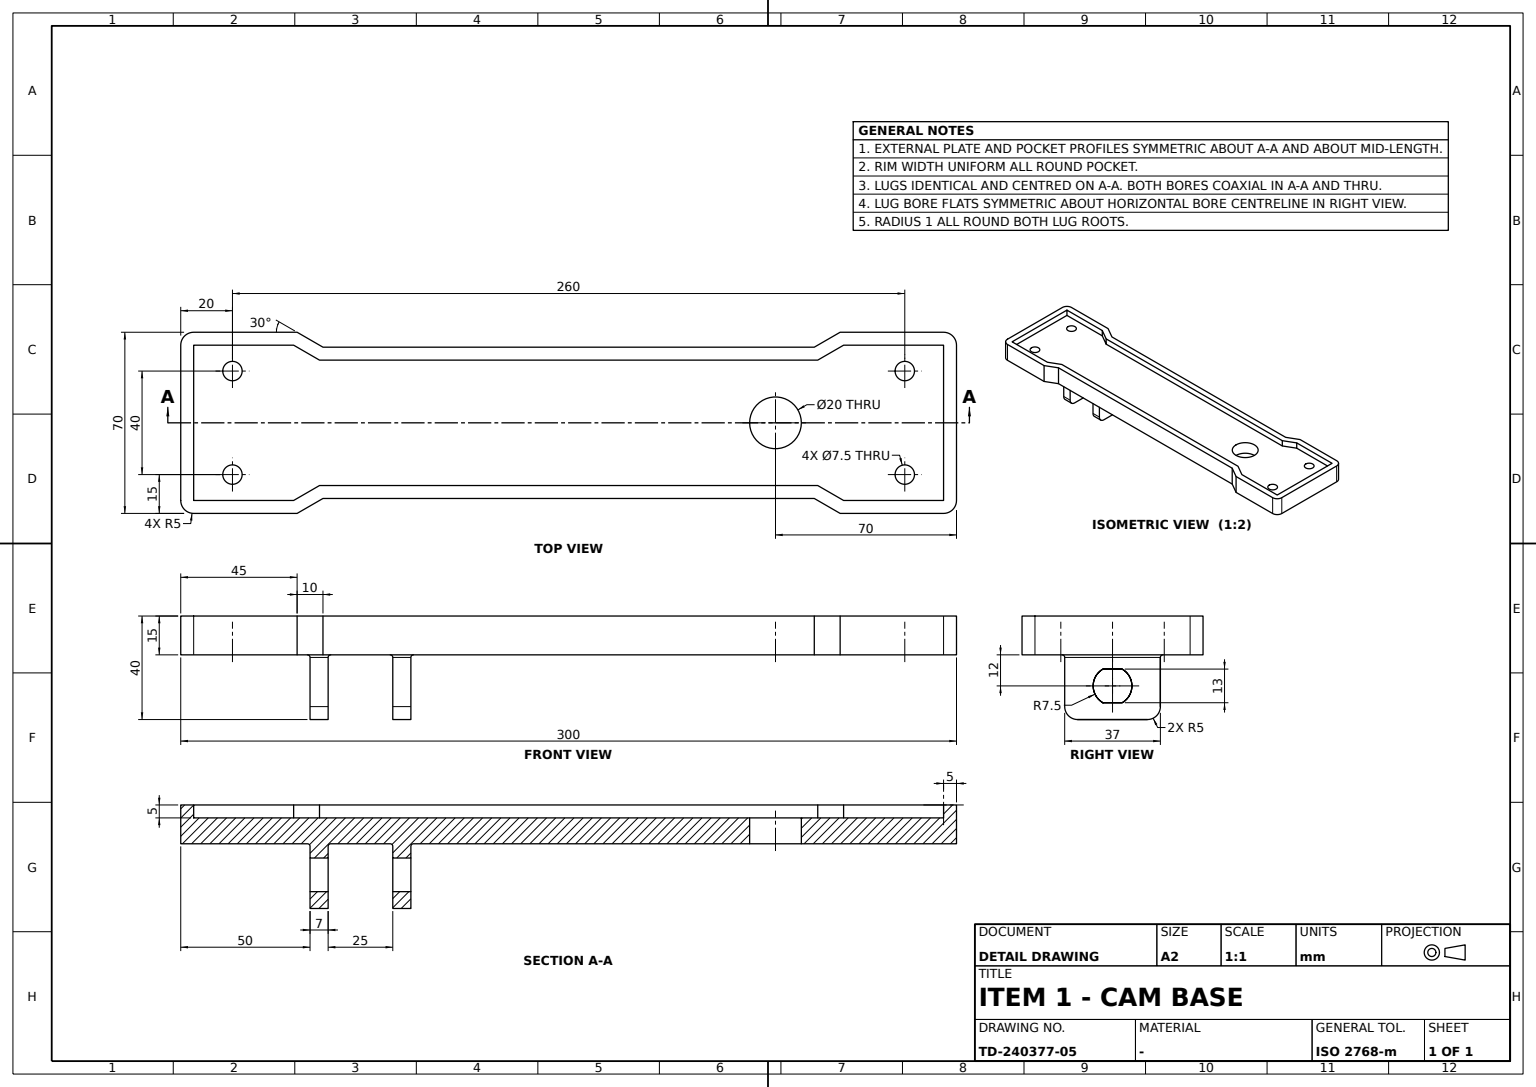
solid
v1 (0,35,105)
v2 (15,35,105)
e1 v1 v2 LINE
v3 (0,35,145)
e2 v3 v1 LINE
v4 (15,35,145)
e3 v3 v4 LINE
e4 v4 v2 LINE
face PLANE(AX(P(0,35,-145),D(0,1,0),D(0,0,1))) [-e1 -e2 e3 e4]
v5 (15,-20,-133.75)
e5 v5 v5 CIRCLE(AX(P(15,-20,-130),D(1,0,0),D(0,0,-1)),3.75)
v6 (5,-20,-126.25)
e6 v6 v6 CIRCLE(AX(P(5,-20,-130),D(-1,0,0),D(0,0,1)),3.75)
face CYL(AX(P(7.5,-20,-130),D(1,0,0),D(0,1,0)),3.75) rev [e5] [e6]
v7 (33.5,3.741657,100)
v8 (20.5,3.741657,100)
e7 v7 v8 CIRCLE(AX(P(27,0,100),D(0,0,-1),D(-1,0,0)),7.5) rev
v9 (20.5,3.741657,93)
e8 v8 v9 LINE
v10 (33.5,3.741657,93)
e9 v10 v9 CIRCLE(AX(P(27,0,93),D(0,0,1),D(1,0,0)),7.5)
e10 v7 v10 LINE
face CYL(AX(P(27,0,-25.66),D(0,0,1),D(1,0,0)),7.5) rev [e7 e8 -e9 -e10]
v11 (16,18.5,93)
v12 (16,18.5,100)
e11 v11 v12 LINE
v13 (15,19.5,92)
e12 v13 v11 ELLIPSE(AX(P(16,19.5,92),D(0,-0.707106781,-0.707106781),D(0,-0.707106781,0.707106781)),1.414214,1) rev
v14 (15,19.5,101)
e13 v13 v14 LINE
e14 v14 v12 ELLIPSE(AX(P(16,19.5,101),D(0,-0.707106781,0.707106781),D(0,0.707106781,0.707106781)),1.414214,1)
face CYL(AX(P(16,19.5,0),D(0,0,1),D(-1,0,0)),1) rev [-e11 -e12 e13 e14]
v15 (15,-19.5,60)
v16 (16,-18.5,61)
e15 v15 v16 ELLIPSE(AX(P(16,-19.5,60),D(0,0.707106781,-0.707106781),D(0,-0.707106781,-0.707106781)),1.414214,1)
v17 (16,-18.5,68)
e16 v17 v16 LINE
v18 (15,-19.5,69)
e17 v18 v17 ELLIPSE(AX(P(16,-19.5,69),D(0,0.707106781,0.707106781),D(0,0.707106781,-0.707106781)),1.414214,1) rev
e18 v18 v15 LINE
face CYL(AX(P(16,-19.5,0),D(0,0,-1),D(-1,0,0)),1) rev [e15 -e16 -e17 e18]
v19 (15,19.5,60)
e19 v19 v15 LINE
v20 (16,18.5,61)
e20 v19 v20 ELLIPSE(AX(P(16,19.5,60),D(0,-0.707106781,-0.707106781),D(0,-0.707106781,0.707106781)),1.414214,1) rev
e21 v20 v16 LINE
face CYL(AX(P(16,0,60),D(0,-1,0),D(-1,0,0)),1) rev [-e15 -e19 e20 e21]
v21 (15,19.5,69)
v22 (16,18.5,68)
e22 v21 v22 ELLIPSE(AX(P(16,19.5,69),D(0,-0.707106781,0.707106781),D(0,0.707106781,0.707106781)),1.414214,1)
e23 v20 v22 LINE
e24 v19 v21 LINE
face CYL(AX(P(16,19.5,0),D(0,0,1),D(-1,0,0)),1) rev [e22 -e23 -e20 e24]
v23 (5,0,-70)
e25 v23 v23 CIRCLE(AX(P(5,0,-80),D(-1,0,0),D(0,0,1)),10)
v24 (15,0,-90)
e26 v24 v24 CIRCLE(AX(P(15,0,-80),D(1,0,0),D(0,0,-1)),10)
face CYL(AX(P(7.5,0,-80),D(1,0,0),D(0,1,0)),10) rev [e25] [e26]
v25 (0,-30,145)
v26 (5,-30,145)
e27 v25 v26 LINE
v27 (0,30,145)
e28 v27 v25 LINE
v28 (5,30,145)
e29 v27 v28 LINE
e30 v28 v26 LINE
face PLANE(AX(P(0,0,145),D(0,0,1),D(0,-1,0))) rev [-e27 -e28 e29 e30]
v29 (15,-29.226497,95)
v30 (15,-29.226497,-95)
e31 v29 v30 LINE
v31 (0,-29.226497,95)
e32 v31 v29 LINE
v32 (0,-29.226497,-95)
e33 v31 v32 LINE
e34 v32 v30 LINE
face PLANE(AX(P(0,-29.226497,95),D(0,-1,0),D(0,0,-1))) [-e31 -e32 e33 e34]
v33 (0,30,150)
e35 v3 v33 CIRCLE(AX(P(0,30,145),D(1,0,0),D(0,0,-1)),5)
v34 (15,30,150)
e36 v33 v34 LINE
e37 v4 v34 CIRCLE(AX(P(15,30,145),D(1,0,0),D(0,0,-1)),5)
face CYL(AX(P(7.5,30,145),D(1,0,0),D(0,1,0)),5) [e35 e36 -e37 -e3]
v35 (15,29.226497,95)
e38 v2 v35 LINE
v36 (0,29.226497,95)
e39 v36 v35 LINE
e40 v1 v36 LINE
face PLANE(AX(P(0,35,105),D(0,-0.866025404,0.5),D(0,-0.5,-0.866025404))) rev [e38 -e39 -e40 e1]
v37 (15,-19.5,101)
e41 v37 v14 LINE
v38 (16,-18.5,100)
e42 v37 v38 ELLIPSE(AX(P(16,-19.5,101),D(0,0.707106781,0.707106781),D(0,0.707106781,-0.707106781)),1.414214,1) rev
e43 v38 v12 LINE
face CYL(AX(P(16,0,101),D(0,1,0),D(-1,0,0)),1) rev [-e41 e42 e43 -e14]
v39 (33.5,-3.741657,100)
v40 (33.5,-3.741657,93)
e44 v39 v40 LINE
e45 v7 v39 LINE
e46 v10 v40 LINE
face PLANE(AX(P(33.5,3.741657,100),D(1,0,0),D(0,-1,0))) rev [-e44 -e45 e10 e46]
v41 (5,20,-126.25)
e47 v41 v41 CIRCLE(AX(P(5,20,-130),D(-1,0,0),D(0,0,1)),3.75)
v42 (5,-20,133.75)
e48 v42 v42 CIRCLE(AX(P(5,-20,130),D(-1,0,0),D(0,0,1)),3.75)
v43 (5,20,133.75)
e49 v43 v43 CIRCLE(AX(P(5,20,130),D(-1,0,0),D(0,0,1)),3.75)
v44 (5,24.226497,96.339746)
v45 (5,30,106.339746)
e50 v44 v45 LINE
v46 (5,24.226497,-96.339746)
e51 v46 v44 LINE
v47 (5,30,-106.339746)
e52 v47 v46 LINE
v48 (5,30,-145)
e53 v48 v47 LINE
v49 (5,-30,-145)
e54 v49 v48 LINE
v50 (5,-30,-106.339746)
e55 v50 v49 LINE
v51 (5,-24.226497,-96.339746)
e56 v51 v50 LINE
v52 (5,-24.226497,96.339746)
e57 v52 v51 LINE
v53 (5,-30,106.339746)
e58 v53 v52 LINE
e59 v26 v53 LINE
e60 v45 v28 LINE
face PLANE(AX(P(5,0,0),D(-1,0,0),D(0,-1,0))) [-e6] [-e25] [-e47] [-e48] [-e49] [-e50 -e51 -e52 -e53 -e54 -e55 -e56 -e57 -e58 -e59 -e30 -e60]
v54 (0,-30,-106.339746)
e61 v54 v50 LINE
v55 (0,-24.226497,-96.339746)
e62 v55 v54 LINE
e63 v55 v51 LINE
face PLANE(AX(P(0,-24.226497,-96.339746),D(0,-0.866025404,0.5),D(0,-0.5,-0.866025404))) rev [-e61 -e62 e63 e56]
v56 (0,24.226497,-96.339746)
e64 v56 v46 LINE
v57 (0,24.226497,96.339746)
e65 v57 v44 LINE
e66 v56 v57 LINE
face PLANE(AX(P(0,24.226497,0),D(0,1,0),D(0,0,1))) rev [e64 e51 -e65 -e66]
v58 (16,-18.5,93)
v59 (35,-18.5,93)
e67 v58 v59 LINE
v60 (35,-18.5,100)
e68 v59 v60 LINE
e69 v38 v60 LINE
e70 v38 v58 LINE
face PLANE(AX(P(15,-18.5,100),D(0,-1,0),D(0,0,-1))) [e67 e68 -e69 e70]
v61 (40,-13.5,68)
v62 (35,-18.5,68)
e71 v61 v62 CIRCLE(AX(P(35,-13.5,68),D(0,0,-1),D(-1,0,0)),5)
v63 (35,-18.5,61)
e72 v63 v62 LINE
v64 (40,-13.5,61)
e73 v63 v64 CIRCLE(AX(P(35,-13.5,61),D(0,0,1),D(1,0,0)),5)
e74 v64 v61 LINE
face CYL(AX(P(35,-13.5,64.5),D(0,0,1),D(0,-1,0)),5) [e71 -e72 e73 e74]
v65 (0,-35,-145)
v66 (0,-35,-105)
e75 v65 v66 LINE
v67 (15,-35,-145)
e76 v65 v67 LINE
v68 (15,-35,-105)
e77 v67 v68 LINE
e78 v66 v68 LINE
face PLANE(AX(P(0,-35,145),D(0,-1,0),D(0,0,-1))) [-e75 e76 e77 -e78]
v69 (33.5,3.741657,61)
v70 (33.5,-3.741657,61)
e79 v69 v70 LINE
v71 (33.5,-3.741657,68)
e80 v71 v70 LINE
v72 (33.5,3.741657,68)
e81 v72 v71 LINE
e82 v72 v69 LINE
face PLANE(AX(P(33.5,3.741657,100),D(1,0,0),D(0,-1,0))) rev [e79 -e80 -e81 e82]
v73 (35,18.5,100)
e83 v12 v73 LINE
v74 (34.999996,18.5,93)
e84 v74 v73 LINE
e85 v11 v74 LINE
face PLANE(AX(P(15,18.5,93),D(0,1,0),D(0,0,1))) [e83 -e84 -e85 e11]
v75 (15,20,-133.75)
e86 v75 v75 CIRCLE(AX(P(15,20,-130),D(1,0,0),D(0,0,-1)),3.75)
face CYL(AX(P(7.5,20,-130),D(1,0,0),D(0,1,0)),3.75) rev [e86] [e47]
v76 (40,13.5,61)
v77 (35,18.5,61)
e87 v76 v77 CIRCLE(AX(P(35,13.5,61),D(0,0,1),D(1,0,0)),5)
e88 v76 v64 LINE
e89 v16 v63 LINE
e90 v20 v77 LINE
v78 (20.5,3.741657,61)
v79 (20.5,-3.741657,61)
e91 v78 v79 LINE
e92 v79 v70 CIRCLE(AX(P(27,0,61),D(0,0,1),D(1,0,0)),7.5)
e93 v69 v78 CIRCLE(AX(P(27,0,61),D(0,0,1),D(1,0,0)),7.5)
face PLANE(AX(P(15,18.5,61),D(0,0,1),D(0,-1,0))) rev [-e87 e88 -e73 -e89 -e21 e90] [e91 e92 -e79 e93]
v80 (20.5,-3.741657,68)
e94 v80 v79 LINE
e95 v71 v80 CIRCLE(AX(P(27,0,68),D(0,0,-1),D(-1,0,0)),7.5)
face CYL(AX(P(27,0,-25.66),D(0,0,1),D(1,0,0)),7.5) rev [-e94 -e95 e80 -e92]
v81 (0,30,-145)
e96 v81 v48 LINE
v82 (0,30,-106.339746)
e97 v82 v47 LINE
e98 v81 v82 LINE
face PLANE(AX(P(0,30,-145),D(0,1,0),D(0,0,1))) rev [e96 e53 -e97 -e98]
v83 (20.5,3.741657,68)
e99 v83 v72 CIRCLE(AX(P(27,0,68),D(0,0,-1),D(-1,0,0)),7.5)
e100 v83 v80 LINE
v84 (35,18.5,68)
e101 v22 v84 LINE
e102 v17 v22 LINE
e103 v17 v62 LINE
v85 (40,13.5,68)
e104 v61 v85 LINE
e105 v84 v85 CIRCLE(AX(P(35,13.5,68),D(0,0,-1),D(-1,0,0)),5)
face PLANE(AX(P(15,-18.5,68),D(0,0,-1),D(0,1,0))) rev [e99 e81 e95 -e100] [-e101 -e102 e103 -e71 e104 -e105]
e106 v76 v85 LINE
face PLANE(AX(P(40,0,0),D(1,0,0),D(0,1,0))) [-e88 e106 -e104 -e74]
v86 (20.5,-3.741657,100)
e107 v86 v39 CIRCLE(AX(P(27,0,100),D(0,0,-1),D(-1,0,0)),7.5) rev
v87 (20.5,-3.741657,93)
e108 v87 v40 CIRCLE(AX(P(27,0,93),D(0,0,1),D(1,0,0)),7.5)
e109 v86 v87 LINE
face CYL(AX(P(27,0,-25.66),D(0,0,1),D(1,0,0)),7.5) rev [e107 e44 -e108 -e109]
v88 (40,-13.5,93)
e110 v59 v88 CIRCLE(AX(P(35,-13.5,93),D(0,0,1),D(1,0,0)),5)
v89 (40,-13.5,100)
e111 v88 v89 LINE
e112 v89 v60 CIRCLE(AX(P(35,-13.5,100),D(0,0,-1),D(-1,0,0)),5)
face CYL(AX(P(35,-13.5,64.5),D(0,0,1),D(0,-1,0)),5) [-e68 e110 e111 e112]
v90 (15,-19.5,92)
e113 v13 v90 LINE
e114 v11 v58 LINE
e115 v90 v58 ELLIPSE(AX(P(16,-19.5,92),D(0,0.707106781,-0.707106781),D(0,-0.707106781,-0.707106781)),1.414214,1)
face CYL(AX(P(16,0,92),D(0,-1,0),D(-1,0,0)),1) rev [-e113 e12 e114 -e115]
v91 (15,30,-150)
v92 (15,35,-145)
e116 v91 v92 CIRCLE(AX(P(15,30,-145),D(1,0,0),D(0,0,-1)),5)
v93 (0,30,-150)
e117 v93 v91 LINE
v94 (0,35,-145)
e118 v93 v94 CIRCLE(AX(P(0,30,-145),D(1,0,0),D(0,0,-1)),5)
e119 v94 v92 LINE
face CYL(AX(P(7.5,30,-145),D(1,0,0),D(0,1,0)),5) [-e116 -e117 e118 e119]
e120 v18 v21 LINE
face CYL(AX(P(16,0,69),D(0,1,0),D(-1,0,0)),1) rev [e102 -e22 -e120 e17]
v95 (0,30,106.339746)
e121 v95 v27 LINE
e122 v95 v45 LINE
face PLANE(AX(P(0,30,-145),D(0,1,0),D(0,0,1))) rev [e60 -e29 -e121 e122]
e123 v57 v95 LINE
face PLANE(AX(P(0,24.226497,96.339746),D(0,0.866025404,-0.5),D(0,0.5,0.866025404))) rev [-e123 e65 e50 -e122]
e124 v83 v78 LINE
face CYL(AX(P(27,0,-25.66),D(0,0,1),D(1,0,0)),7.5) rev [-e99 e124 -e93 -e82]
v96 (0,-24.226497,96.339746)
e125 v96 v55 LINE
e126 v96 v52 LINE
face PLANE(AX(P(0,-24.226497,0),D(0,-1,0),D(0,0,-1))) rev [-e125 e126 e57 -e63]
v97 (0,35,-105)
v98 (0,29.226497,-95)
e127 v97 v98 LINE
v99 (15,29.226497,-95)
e128 v98 v99 LINE
v100 (15,35,-105)
e129 v100 v99 LINE
e130 v97 v100 LINE
face PLANE(AX(P(0,35,-105),D(0,0.866025404,0.5),D(0,-0.5,0.866025404))) [e127 e128 -e129 -e130]
v101 (40,13.5,100)
e131 v89 v101 LINE
v102 (40,13.5,93)
e132 v102 v88 LINE
e133 v102 v101 LINE
face PLANE(AX(P(40,0,0),D(1,0,0),D(0,1,0))) [-e131 -e111 -e132 e133]
e134 v102 v74 CIRCLE(AX(P(35,13.5,93),D(0,0,1),D(1,0,0)),5)
e135 v9 v87 LINE
face PLANE(AX(P(15,18.5,93),D(0,0,1),D(0,-1,0))) rev [e132 -e110 -e67 -e114 e85 -e134] [e9 e135 e108 -e46]
e136 v82 v56 LINE
face PLANE(AX(P(0,30,-106.339746),D(0,0.866025404,0.5),D(0,-0.5,0.866025404))) rev [-e64 -e136 e97 e52]
e137 v94 v97 LINE
e138 v92 v100 LINE
face PLANE(AX(P(0,35,-145),D(0,1,0),D(0,0,1))) [-e119 e137 e130 -e138]
e139 v37 v90 LINE
face CYL(AX(P(16,-19.5,0),D(0,0,-1),D(-1,0,0)),1) rev [-e42 e139 e115 -e70]
v103 (0,-30,-150)
v104 (15,-30,-150)
e140 v103 v104 LINE
e141 v67 v104 CIRCLE(AX(P(15,-30,-145),D(1,0,0),D(0,0,-1)),5)
e142 v65 v103 CIRCLE(AX(P(0,-30,-145),D(1,0,0),D(0,0,-1)),5)
face CYL(AX(P(7.5,-30,-145),D(1,0,0),D(0,1,0)),5) [e140 -e141 -e76 e142]
e143 v73 v101 CIRCLE(AX(P(35,13.5,100),D(0,0,-1),D(-1,0,0)),5)
face CYL(AX(P(35,13.5,64.5),D(0,0,1),D(0,1,0)),5) [e134 e84 e143 -e133]
e144 v66 v32 LINE
e145 v68 v30 LINE
face PLANE(AX(P(0,-35,-105),D(0,0.866025404,-0.5),D(0,0.5,0.866025404))) rev [-e144 e78 e145 -e34]
e146 v98 v36 LINE
e147 v93 v103 LINE
v105 (0,-35,105)
e148 v105 v31 LINE
v106 (0,-35,145)
e149 v106 v105 LINE
v107 (0,-30,150)
e150 v107 v106 CIRCLE(AX(P(0,-30,145),D(1,0,0),D(0,0,-1)),5)
e151 v33 v107 LINE
v108 (0,-30,106.339746)
e152 v25 v108 LINE
e153 v108 v96 LINE
v109 (0,-30,-145)
e154 v54 v109 LINE
e155 v109 v81 LINE
face PLANE(AX(P(0,0,0),D(1,0,0),D(0,1,0))) rev [e40 -e146 -e127 -e137 -e118 e147 -e142 e75 e144 -e33 -e148 -e149 -e150 -e151 -e35 e2] [e28 e152 e153 e125 e62 e154 e155 e98 e136 e66 e123 e121]
v110 (15,20,126.25)
e156 v110 v110 CIRCLE(AX(P(15,20,130),D(1,0,0),D(0,0,-1)),3.75)
v111 (15,-20,126.25)
e157 v111 v111 CIRCLE(AX(P(15,-20,130),D(1,0,0),D(0,0,-1)),3.75)
e158 v91 v104 LINE
e159 v99 v35 LINE
v112 (15,-30,150)
e160 v34 v112 LINE
v113 (15,-35,145)
e161 v112 v113 CIRCLE(AX(P(15,-30,145),D(1,0,0),D(0,0,-1)),5)
v114 (15,-35,105)
e162 v113 v114 LINE
e163 v114 v29 LINE
face PLANE(AX(P(15,0,0),D(1,0,0),D(0,1,0))) [e120 -e24 e19 -e18] [-e156] [-e157] [-e86] [-e145 -e77 e141 -e158 e116 e138 e129 e159 -e38 -e4 e37 e160 e161 e162 e163 e31] [e41 -e13 e113 -e139] [-e5] [-e26]
e164 v107 v112 LINE
face PLANE(AX(P(0,0,150),D(0,0,1),D(0,-1,0))) [-e36 e151 e164 -e160]
e165 v105 v114 LINE
face PLANE(AX(P(0,-35,105),D(0,-0.866025404,-0.5),D(0,0.5,-0.866025404))) [e32 -e163 -e165 e148]
face CYL(AX(P(7.5,-20,130),D(1,0,0),D(0,1,0)),3.75) rev [e157] [e48]
e166 v77 v84 LINE
face PLANE(AX(P(15,18.5,93),D(0,1,0),D(0,0,1))) [-e166 -e90 e23 e101]
e167 v108 v53 LINE
face PLANE(AX(P(0,-30,106.339746),D(0,-0.866025404,-0.5),D(0,0.5,-0.866025404))) rev [-e126 -e153 e167 e58]
face PLANE(AX(P(15,-18.5,100),D(0,-1,0),D(0,0,-1))) [e89 e72 -e103 e16]
e168 v8 v86 LINE
face PLANE(AX(P(15,-18.5,100),D(0,0,-1),D(0,1,0))) rev [e45 -e107 -e168 -e7] [-e43 e69 -e112 e131 -e143 -e83]
face CYL(AX(P(35,13.5,64.5),D(0,0,1),D(0,1,0)),5) [e87 e166 e105 -e106]
e169 v106 v113 LINE
face CYL(AX(P(7.5,-30,145),D(1,0,0),D(0,1,0)),5) [e169 -e161 -e164 e150]
face PLANE(AX(P(0,-30,-106.339746),D(0,-1,0),D(0,0,-1))) rev [-e152 e27 e59 -e167]
face CYL(AX(P(7.5,20,130),D(1,0,0),D(0,1,0)),3.75) rev [e156] [e49]
e170 v109 v49 LINE
face PLANE(AX(P(0,-30,-106.339746),D(0,-1,0),D(0,0,-1))) rev [-e154 e61 e55 -e170]
face PLANE(AX(P(0,0,-145),D(0,0,-1),D(0,1,0))) rev [e54 -e96 -e155 e170]
face PLANE(AX(P(20.5,3.741657,100),D(1,0,0),D(0,-1,0))) [e94 -e91 -e124 e100]
face PLANE(AX(P(20.5,3.741657,100),D(1,0,0),D(0,-1,0))) [-e8 e168 e109 -e135]
face PLANE(AX(P(0,0,-150),D(0,0,1),D(0,-1,0))) rev [e158 -e140 -e147 e117]
face PLANE(AX(P(0,-35,145),D(0,-1,0),D(0,0,-1))) [-e169 e149 e165 -e162]
face PLANE(AX(P(0,29.226497,-95),D(0,1,0),D(0,0,1))) [-e159 -e128 e146 e39]
